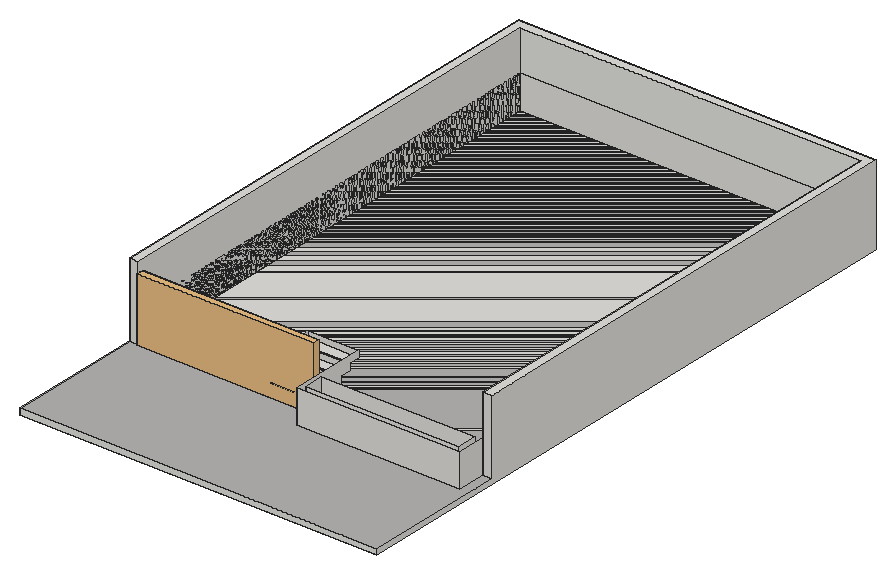
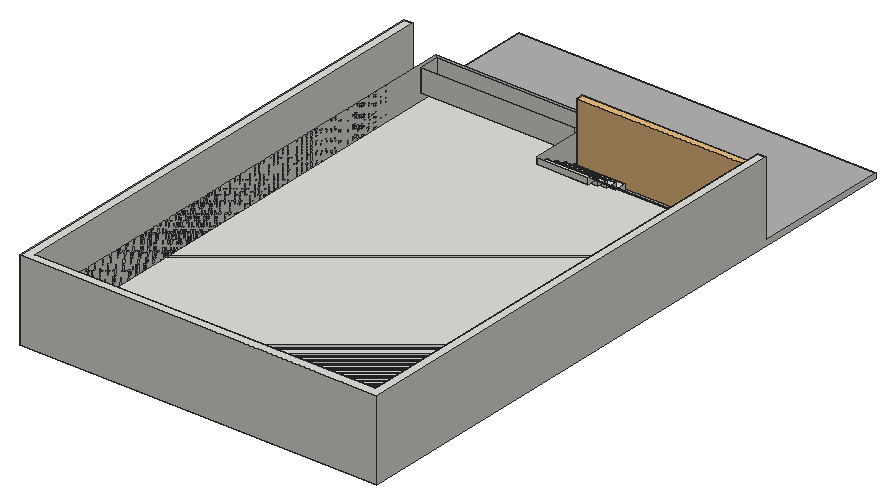
# SketchUp Ruby script. Lengths in inches.
U = 1.inch
M = Sketchup.active_model
def pt(a) = Geom::Point3d.new(a.map { |v| v * U })
def face(e, loops, mat)
  f = e.add_face(loops[0].map { |a| pt(a) })
  loops[1..].each { |l| e.add_face(l.map { |a| pt(a) }).erase! }
  f.material = f.back_material = mat if mat
  f
end
# faces: each face lists its corners as indices into pts; further lists are holes
def faces(e, pts, list, mat = nil) = list.each { |f| face(e, (f[0].is_a?(Array) ? f : [f]).map { |l| l.map { |i| pts[i] } }, mat) }
# xy, xz, yz: faces in a plane at the given z, y or x. An outline is a flat list of corners, or four numbers for a rectangle; further outlines are holes
def ring(l) = l.size == 4 ? [[l[0], l[1]], [l[2], l[1]], [l[2], l[3]], [l[0], l[3]]] : l.each_slice(2).to_a
def flat(e, list, mat, &to3) = list.each { |f| face(e, (f[0].is_a?(Array) ? f : [f]).map { |l| ring(l).map { |u, v| to3.(u, v) } }, mat) }
def xy(e, z, list, mat = nil) = flat(e, list, mat) { |x, y| [x, y, z] }
def xz(e, y, list, mat = nil) = flat(e, list, mat) { |x, z| [x, y, z] }
def yz(e, x, list, mat = nil) = flat(e, list, mat) { |y, z| [x, y, z] }
def lines(e, pts, list) = list.each { |a, b| e.add_line(pt(pts[a]), pt(pts[b])) }
# prism: a flat outline (further loops are holes) pulled along v
def prism(e, loops, v, mat = nil)
  f = face(e, loops, mat); d = Geom::Vector3d.new(v.map { |x| x * U })
  f.pushpull(f.normal.samedirection?(d) ? d.length : -d.length)
end
def box(e, o, s, mat = nil) = prism(e, [[o, [o[0] + s[0], o[1], o[2]], [o[0] + s[0], o[1] + s[1], o[2]], [o[0], o[1] + s[1], o[2]]]], [0, 0, s[2]], mat)
def at(x, y, z, deg = 0) = Geom::Transformation.translation(pt([x, y, z])) * Geom::Transformation.rotation(ORIGIN, Z_AXIS, deg.degrees)
def axes(o, x, y, z) = Geom::Transformation.new([*x, 0, *y, 0, *z, 0, *pt(o).to_a, 1])
def part(name) = M.definitions.add(name)
# library, detail: a bought-in or finely detailed component or shape, given as its bounding box
def library(name, o, s) = part(name).tap { |d| box(d.entities, o, s) }
def detail(e, o, s) = box(e.add_group.entities, o, s)
def put(e, d, t, mat = nil) = e.add_instance(d, t).tap { |i| i.material = mat if mat }
def group(e, t, mat = nil) = e.add_group.tap { |g| g.transformation = t; g.material = mat if mat }.entities
root = M.entities
M.materials.add("[Formica Graystone]").color = [224, 223, 219]
M.materials.add("[Granite Tile]").color = [182, 180, 179]
c1 = library("Metal mesh gate",[0,-1.63,0],[123.41,6.81,51.8125])
xy(root,-5.18,[[195,120,195,153,9,153,9,645,366,645,366,120]],"[Formica Graystone]")
xy(root,-2.3,[[9,157.12,141,157.37]],"[Formica Graystone]")
xy(root,0.82,[[141,152.95,195,153]],"[Formica Graystone]")
xy(root,1.24,[[9,161.97,141,162.22]],"[Formica Graystone]")
xy(root,1.82,[[141,152.95,195,153],[141,153,195,165]],"[Formica Graystone]")
xy(root,4.77,[[9,166.8125,141,167.0625]],"[Formica Graystone]")
xy(root,6.82,[[200,125,361,145]],"[Formica Graystone]")
xy(root,7.82,[[141,164.95,195,165]],"[Formica Graystone]")
xy(root,8.31,[[9,171.66,141,171.91]],"[Formica Graystone]")
xy(root,8.82,[[141,164.95,195,165],[141,165,195,177]],"[Formica Graystone]")
xy(root,11.84,[[9,176.51,141,176.76]],"[Formica Graystone]")
xy(root,14.82,[[141,176.95,195,177]],"[Formica Graystone]")
xy(root,15.38,[[9,181.36,141,181.61]],"[Formica Graystone]")
xy(root,15.82,[[141,176.95,195,177],[141,177,195,189]],"[Formica Graystone]")
xy(root,18.91,[[9,186.21,141,186.46]],"[Formica Graystone]")
xy(root,21.82,[[141,188.95,195,189]],"[Formica Graystone]")
xy(root,22.45,[[9,191.05,141,191.3]],"[Formica Graystone]")
xy(root,22.82,[[141,188.95,195,189],[141,189,195,201]],"[Formica Graystone]")
xz(root,120,[[195,-5.18,366,29.82]],"[Formica Graystone]")
xz(root,125,[[200,6.82,361,30.82]],"[Formica Graystone]")
xz(root,145,[[200,6.82,361,30.82]],"[Formica Graystone]")
xz(root,152.5,[[141,1.27,195,1.32],[141,1.32,195,1.37]],"[Formica Graystone]")
xz(root,153,[[141,-5.18,195,0.82]],"[Formica Graystone]")
xz(root,157.12,[[9,-2.3,141,-2.18]],"[Formica Graystone]")
xz(root,157.37,[[9,-2.3,141,-2]],"[Formica Graystone]")
xz(root,161.97,[[9,1.24,141,1.36]],"[Formica Graystone]")
xz(root,162.22,[[9,1.24,141,1.54]],"[Formica Graystone]")
xz(root,164.5,[[141,8.27,195,8.32],[141,8.32,195,8.37]],"[Formica Graystone]")
xz(root,165,[[141,1.82,195,7.82]],"[Formica Graystone]")
xz(root,166.8125,[[9,4.77,141,4.89]],"[Formica Graystone]")
xz(root,167.0625,[[9,4.77,141,5.07]],"[Formica Graystone]")
xz(root,171.66,[[9,8.31,141,8.43]],"[Formica Graystone]")
xz(root,171.91,[[9,8.31,141,8.61]],"[Formica Graystone]")
xz(root,176.5,[[141,15.27,195,15.32],[141,15.32,195,15.37]],"[Formica Graystone]")
xz(root,176.51,[[9,11.84,141,11.96]],"[Formica Graystone]")
xz(root,176.76,[[9,11.84,141,12.14]],"[Formica Graystone]")
xz(root,177,[[141,8.82,195,14.82]],"[Formica Graystone]")
xz(root,181.36,[[9,15.38,141,15.5]],"[Formica Graystone]")
xz(root,181.61,[[9,15.38,141,15.68]],"[Formica Graystone]")
xz(root,186.21,[[9,18.91,141,19.03]],"[Formica Graystone]")
xz(root,186.46,[[9,18.91,141,19.21]],"[Formica Graystone]")
xz(root,188.5,[[141,22.27,195,22.32],[141,22.32,195,22.37]],"[Formica Graystone]")
xz(root,189,[[141,15.82,195,21.82]],"[Formica Graystone]")
xz(root,191.05,[[9,22.45,141,22.57]],"[Formica Graystone]")
xz(root,191.3,[[9,22.45,141,22.75]],"[Formica Graystone]")
xz(root,201,[[141,22.82,195,28.82]],"[Formica Graystone]")
xz(root,645,[[9,-5.18,366,29.82]],"[Formica Graystone]")
yz(root,9,[[153,-5.18,157.12,-2.18,157.12,-2.3,157.37,-2.3,157.37,-2,161.97,1.36,161.97,1.24,162.22,1.24,162.22,1.54,166.8125,4.89,166.8125,4.77,167.0625,4.77,167.0625,5.07,171.66,8.43,171.66,8.31,171.91,8.31,171.91,8.61,176.51,11.96,176.51,11.84,176.76,11.84,176.76,12.14,181.36,15.5,181.36,15.38,181.61,15.38,181.61,15.68,186.21,19.03,186.21,18.91,186.46,18.91,186.46,19.21,191.05,22.57,191.05,22.45,191.3,22.45,191.3,22.75,195.9,26.1,195.9,25.98,196.15,25.98,196.15,26.28,201,29.82,645,29.82,645,-5.18]],"[Formica Graystone]")
yz(root,141,[[153,-5.18,153,0.82,152.95,0.82,152.85,0.84,152.8,0.86,152.75,0.89,152.71,0.91,152.67,0.95,152.63,0.98,152.6,1.03,152.57,1.07,152.54,1.12,152.52,1.16,152.51,1.22,152.5,1.27,152.5,1.37,152.52,1.47,152.54,1.52,152.57,1.57,152.63,1.65,152.67,1.69,152.75,1.75,152.8,1.78,152.85,1.79,152.9,1.81,152.95,1.82,162.6,1.82,162.22,1.54,162.22,1.24,161.97,1.24,161.97,1.36,157.37,-2,157.37,-2.3,157.12,-2.3,157.12,-2.18],[162.6,1.82,165,1.82,165,3.57],[165,3.57,165,7.82,164.95,7.82,164.85,7.84,164.8,7.86,164.75,7.89,164.71,7.91,164.67,7.95,164.63,7.98,164.6,8.03,164.57,8.07,164.54,8.12,164.52,8.16,164.51,8.22,164.5,8.27,164.5,8.37,164.52,8.47,164.54,8.52,164.57,8.57,164.63,8.65,164.67,8.69,164.75,8.75,164.8,8.78,164.85,8.79,164.9,8.81,164.95,8.82,172.2,8.82,171.91,8.61,171.91,8.31,171.66,8.31,171.66,8.43,167.0625,5.07,167.0625,4.77,166.8125,4.77,166.8125,4.89],[172.2,8.82,177,8.82,177,12.32,176.76,12.14,176.76,11.84,176.51,11.84,176.51,11.96],[177,12.32,177,14.82,176.95,14.82,176.85,14.84,176.8,14.86,176.75,14.89,176.71,14.91,176.67,14.95,176.63,14.98,176.6,15.03,176.57,15.07,176.54,15.12,176.52,15.16,176.51,15.22,176.5,15.27,176.5,15.37,176.52,15.47,176.54,15.52,176.57,15.57,176.63,15.65,176.67,15.69,176.75,15.75,176.8,15.78,176.85,15.79,176.9,15.81,176.95,15.82,181.8,15.82,181.61,15.68,181.61,15.38,181.36,15.38,181.36,15.5],
  [181.8,15.82,189,15.82,189,21.07,186.46,19.21,186.46,18.91,186.21,18.91,186.21,19.03],[189,21.07,189,21.82,188.95,21.82,188.85,21.84,188.8,21.86,188.75,21.89,188.71,21.91,188.67,21.95,188.63,21.98,188.6,22.03,188.57,22.07,188.54,22.12,188.52,22.16,188.51,22.22,188.5,22.27,188.5,22.37,188.52,22.47,188.54,22.52,188.57,22.57,188.63,22.65,188.67,22.69,188.75,22.75,188.8,22.78,188.85,22.79,188.9,22.81,188.95,22.82,191.4,22.82,191.3,22.75,191.3,22.45,191.05,22.45,191.05,22.57],[191.4,22.82,201,22.82,201,28.82,200.95,28.82,200.85,28.84,200.8,28.86,200.75,28.89,200.71,28.91,200.67,28.95,200.63,28.98,200.6,29.03,200.57,29.07,200.54,29.12,200.52,29.16,200.51,29.22,200.5,29.27,200.5,29.37,200.52,29.47,196.15,26.28,196.15,25.98,195.9,25.98,195.9,26.1]],"[Formica Graystone]")
yz(root,195,[[120,-5.18,120,29.82,201,29.82,200.95,29.82,200.9,29.81,200.85,29.79,200.8,29.78,200.75,29.75,200.67,29.69,200.63,29.65,200.57,29.57,200.54,29.52,200.52,29.47,200.5,29.37,200.5,29.27,200.51,29.22,200.52,29.16,200.54,29.12,200.57,29.07,200.6,29.03,200.63,28.98,200.67,28.95,200.71,28.91,200.75,28.89,200.8,28.86,200.85,28.84,200.95,28.82,201,28.82,201,22.82,188.95,22.82,188.9,22.81,188.85,22.79,188.8,22.78,188.75,22.75,188.67,22.69,188.63,22.65,188.57,22.57,188.54,22.52,188.52,22.47,188.5,22.37,188.5,22.27,188.51,22.22,188.52,22.16,188.54,22.12,188.57,22.07,188.6,22.03,188.63,21.98,188.67,21.95,188.71,21.91,188.75,21.89,188.8,21.86,188.85,21.84,188.95,21.82,189,21.82,189,15.82,176.95,15.82,176.9,15.81,176.85,15.79,176.8,15.78,176.75,15.75,176.67,15.69,176.63,15.65,176.57,15.57,176.54,15.52,176.52,15.47,176.5,15.37,176.5,15.27,176.51,15.22,176.52,15.16,176.54,15.12,176.57,15.07,176.6,15.03,176.63,14.98,176.67,14.95,176.71,14.91,176.75,14.89,176.8,14.86,176.85,14.84,176.95,14.82,177,14.82,177,8.82,164.95,8.82,164.9,8.81,164.85,8.79,164.8,8.78,164.75,8.75,164.67,8.69,164.63,8.65,164.57,8.57,164.54,8.52,164.52,8.47,164.5,8.37,164.5,8.27,164.51,8.22,164.52,8.16,164.54,8.12,164.57,8.07,164.6,8.03,164.63,7.98,164.67,7.95,164.71,7.91,164.75,7.89,164.8,7.86,164.85,7.84,164.95,7.82,165,7.82,165,1.82,152.95,1.82,152.9,1.81,152.85,1.79,152.8,1.78,152.75,1.75,152.67,1.69,152.63,1.65,152.57,1.57,152.54,1.52,152.52,1.47,152.5,1.37,152.5,1.27,152.51,1.22,152.52,1.16,152.54,1.12,152.57,1.07,152.6,1.03,152.63,0.98,152.67,0.95,152.71,0.91,152.75,0.89,152.8,0.86,152.85,0.84,152.95,0.82,153,0.82,153,-5.18]],"[Formica Graystone]")
yz(root,200,[[125,6.82,145,30.82]],"[Formica Graystone]")
yz(root,361,[[125,6.82,145,30.82]],"[Formica Graystone]")
yz(root,366,[[120,-5.18,645,29.82]],"[Formica Graystone]")
p = [[141,153,-5.18],[141,157.12,-2.18],[9,157.12,-2.18],[9,153,-5.18],[141,157.37,-2],[141,161.97,1.36],
  [9,161.97,1.36],[9,157.37,-2],[195,152.9,0.83],[195,152.85,0.84],[141,152.85,0.84],[141,152.9,0.83],
  [195,152.8,0.86],[141,152.8,0.86],[195,152.95,0.82],[141,152.95,0.82],[195,152.67,0.95],[195,152.63,0.98],
  [141,152.63,0.98],[141,152.67,0.95],[195,152.75,0.89],[195,152.71,0.91],[141,152.71,0.91],[141,152.75,0.89],
  [195,152.6,1.03],[141,152.6,1.03],[195,152.57,1.07],[141,152.57,1.07],[195,152.54,1.12],[141,152.54,1.12],
  [195,152.52,1.16],[141,152.52,1.16],[195,152.51,1.22],[141,152.51,1.22],[195,152.5,1.27],[141,152.5,1.27],
  [195,152.5,1.37],[195,152.51,1.42],[141,152.51,1.42],[141,152.5,1.37],[195,152.52,1.47],[141,152.52,1.47],
  [195,152.54,1.52],[141,152.54,1.52],[195,152.57,1.57],[141,152.57,1.57],[141,162.22,1.54],[141,162.6,1.82],
  [141,165,3.57],[141,166.8125,4.89],[9,166.8125,4.89],[9,162.22,1.54],[195,152.6,1.61],[141,152.6,1.61],
  [195,152.63,1.65],[141,152.63,1.65],[195,152.67,1.69],[141,152.67,1.69],[195,152.71,1.72],[141,152.71,1.72],
  [195,152.75,1.75],[141,152.75,1.75],[195,152.8,1.78],[141,152.8,1.78],[195,152.85,1.79],[141,152.85,1.79],
  [195,152.9,1.81],[141,152.9,1.81],[195,152.95,1.82],[141,152.95,1.82],[141,167.0625,5.07],[141,171.66,8.43],
  [9,171.66,8.43],[9,167.0625,5.07],[195,164.9,7.83],[195,164.85,7.84],[141,164.85,7.84],[141,164.9,7.83],
  [195,164.8,7.86],[141,164.8,7.86],[195,164.95,7.82],[141,164.95,7.82],[195,164.67,7.95],[195,164.63,7.98],
  [141,164.63,7.98],[141,164.67,7.95],[195,164.75,7.89],[195,164.71,7.91],[141,164.71,7.91],[141,164.75,7.89],
  [195,164.6,8.03],[141,164.6,8.03],[195,164.57,8.07],[141,164.57,8.07],[195,164.54,8.12],[141,164.54,8.12],
  [195,164.52,8.16],[141,164.52,8.16],[195,164.51,8.22],[141,164.51,8.22],[195,164.5,8.27],[141,164.5,8.27],
  [195,164.5,8.37],[195,164.51,8.42],[141,164.51,8.42],[141,164.5,8.37],[195,164.52,8.47],[141,164.52,8.47],
  [195,164.54,8.52],[141,164.54,8.52],[195,164.57,8.57],[141,164.57,8.57],[195,164.6,8.61],[141,164.6,8.61],
  [195,164.63,8.65],[141,164.63,8.65],[141,171.91,8.61],[141,172.2,8.82],[141,176.51,11.96],[9,176.51,11.96],
  [9,171.91,8.61],[195,164.67,8.69],[141,164.67,8.69],[195,164.71,8.72],[141,164.71,8.72],[195,164.75,8.75],
  [141,164.75,8.75],[195,164.8,8.78],[141,164.8,8.78],[195,164.85,8.79],[141,164.85,8.79],[195,164.9,8.81],
  [141,164.9,8.81],[195,164.95,8.82],[141,164.95,8.82],[141,176.76,12.14],[141,177,12.32],[141,181.36,15.5],
  [9,181.36,15.5],[9,176.76,12.14],[195,176.9,14.83],[195,176.85,14.84],[141,176.85,14.84],[141,176.9,14.83],
  [195,176.8,14.86],[141,176.8,14.86],[195,176.95,14.82],[141,176.95,14.82],[195,176.67,14.95],[195,176.63,14.98],
  [141,176.63,14.98],[141,176.67,14.95],[195,176.75,14.89],[195,176.71,14.91],[141,176.71,14.91],[141,176.75,14.89],
  [195,176.6,15.03],[141,176.6,15.03],[195,176.57,15.07],[141,176.57,15.07],[195,176.54,15.12],[141,176.54,15.12],
  [195,176.52,15.16],[141,176.52,15.16],[195,176.51,15.22],[141,176.51,15.22],[195,176.5,15.27],[141,176.5,15.27],
  [195,176.5,15.37],[195,176.51,15.42],[141,176.51,15.42],[141,176.5,15.37],[195,176.52,15.47],[141,176.52,15.47],
  [195,176.54,15.52],[141,176.54,15.52],[195,176.57,15.57],[141,176.57,15.57],[195,176.6,15.61],[141,176.6,15.61],
  [195,176.63,15.65],[141,176.63,15.65],[195,176.67,15.69],[141,176.67,15.69],[195,176.71,15.72],[141,176.71,15.72],
  [195,176.75,15.75],[141,176.75,15.75],[141,181.61,15.68],[141,181.8,15.82],[141,186.21,19.03],[9,186.21,19.03],
  [9,181.61,15.68],[195,176.8,15.78],[141,176.8,15.78],[195,176.85,15.79],[141,176.85,15.79],[195,176.9,15.81],
  [141,176.9,15.81],[195,176.95,15.82],[141,176.95,15.82],[141,186.46,19.21],[141,189,21.07],[141,191.05,22.57],
  [9,191.05,22.57],[9,186.46,19.21],[195,188.9,21.83],[195,188.85,21.84],[141,188.85,21.84],[141,188.9,21.83],
  [195,188.8,21.86],[141,188.8,21.86],[195,188.95,21.82],[141,188.95,21.82],[195,188.67,21.95],[195,188.63,21.98],
  [141,188.63,21.98],[141,188.67,21.95],[195,188.75,21.89],[195,188.71,21.91],[141,188.71,21.91],[141,188.75,21.89],
  [195,188.6,22.03],[141,188.6,22.03],[195,188.57,22.07],[141,188.57,22.07],[195,188.54,22.12],[141,188.54,22.12],
  [195,188.52,22.16],[141,188.52,22.16],[195,188.51,22.22],[141,188.51,22.22],[195,188.5,22.27],[141,188.5,22.27],
  [195,188.5,22.37],[195,188.51,22.42],[141,188.51,22.42],[141,188.5,22.37],[195,188.52,22.47],[141,188.52,22.47],
  [195,188.54,22.52],[141,188.54,22.52],[195,188.57,22.57],[141,188.57,22.57],[195,188.6,22.61],[141,188.6,22.61],
  [195,188.63,22.65],[141,188.63,22.65],[195,188.67,22.69],[141,188.67,22.69],[195,188.71,22.72],[141,188.71,22.72],
  [195,188.75,22.75],[141,188.75,22.75],[141,191.3,22.75],[141,191.4,22.82],[141,195.9,26.1],[9,195.9,26.1],
  [9,191.3,22.75],[195,188.8,22.78],[141,188.8,22.78],[195,188.85,22.79],[141,188.85,22.79],[195,188.9,22.81],
  [141,188.9,22.81],[195,188.95,22.82],[141,188.95,22.82]]
faces(root,p,[[0,1,2,3],[4,5,6,7],[8,9,10,11],[9,12,13,10],[14,8,11,15],[16,17,18,19],[20,21,22,23],[21,16,19,22],
  [12,20,23,13],[17,24,25,18],[24,26,27,25],[26,28,29,27],[28,30,31,29],[30,32,33,31],[32,34,35,33],[36,37,38,39],
  [37,40,41,38],[40,42,43,41],[42,44,45,43],[46,47,48,49,50,51],[44,52,53,45],[52,54,55,53],[54,56,57,55],[56,58,59,57],
  [58,60,61,59],[60,62,63,61],[62,64,65,63],[64,66,67,65],[66,68,69,67],[70,71,72,73],[74,75,76,77],[75,78,79,76],
  [80,74,77,81],[82,83,84,85],[86,87,88,89],[87,82,85,88],[78,86,89,79],[83,90,91,84],[90,92,93,91],[92,94,95,93],
  [94,96,97,95],[96,98,99,97],[98,100,101,99],[102,103,104,105],[103,106,107,104],[106,108,109,107],[108,110,111,109],[110,112,113,111],
  [112,114,115,113],[116,117,118,119,120],[114,121,122,115],[121,123,124,122],[123,125,126,124],[125,127,128,126],[127,129,130,128],[129,131,132,130],
  [131,133,134,132],[135,136,137,138,139],[140,141,142,143],[141,144,145,142],[146,140,143,147],[148,149,150,151],[152,153,154,155],[153,148,151,154],
  [144,152,155,145],[149,156,157,150],[156,158,159,157],[158,160,161,159],[160,162,163,161],[162,164,165,163],[164,166,167,165],[168,169,170,171],
  [169,172,173,170],[172,174,175,173],[174,176,177,175],[176,178,179,177],[178,180,181,179],[180,182,183,181],[182,184,185,183],[184,186,187,185],
  [188,189,190,191,192],[186,193,194,187],[193,195,196,194],[195,197,198,196],[197,199,200,198],[201,202,203,204,205],[206,207,208,209],[207,210,211,208],
  [212,206,209,213],[214,215,216,217],[218,219,220,221],[219,214,217,220],[210,218,221,211],[215,222,223,216],[222,224,225,223],[224,226,227,225],
  [226,228,229,227],[228,230,231,229],[230,232,233,231],[234,235,236,237],[235,238,239,236],[238,240,241,239],[240,242,243,241],[242,244,245,243],
  [244,246,247,245],[246,248,249,247],[248,250,251,249],[250,252,253,251],[254,255,256,257,258],[252,259,260,253],[259,261,262,260],[261,263,264,262],
  [263,265,266,264]],"[Formica Graystone]")
g1 = group(root,at(9,120,-5.18))
xy(g1,-6,[[-9,-120,366,534]])
xy(g1,0,[[-9,-120,366,-120,366,30,357,30,357,525,0,525,0,24,-9,24]],"[Granite Tile]")
xy(g1,78,[[-9,24,0,24,0,525,357,525,357,30,366,30,366,534,-9,534]],"[Formica Graystone]")
xz(g1,-120,[[-9,-6,366,0]])
xz(g1,24,[[-9,0,0,78]],"[Formica Graystone]")
xz(g1,30,[[357,0,366,78]],"[Formica Graystone]")
xz(g1,525,[[0,0,357,78]])
xz(g1,534,[[-9,-6,366,78]])
yz(g1,-9,[[-120,-6,-120,0,24,0,24,78,534,78,534,-6]])
yz(g1,0,[[24,0,525,78]],"[Formica Graystone]")
yz(g1,357,[[30,0,525,78]])
yz(g1,366,[[-120,-6,534,-6,534,78,30,78,30,0,-120,0]],"[Formica Graystone]")
put(root,c1,axes([9,144,-5.18],[1.5,0,0],[0,1,0],[0,0,1.3]))
